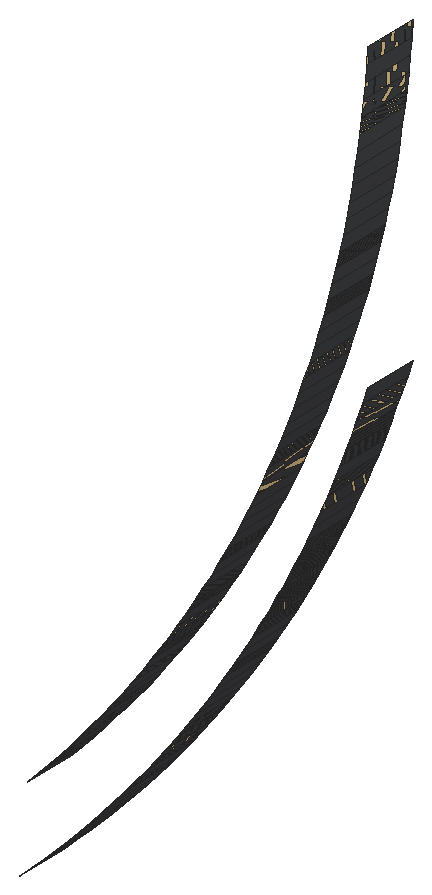
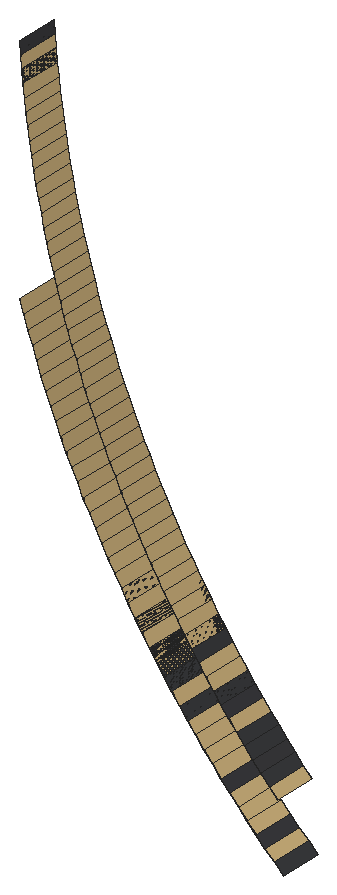
# SketchUp Ruby script. Lengths in inches.
U = 1.inch
M = Sketchup.active_model
def pt(a) = Geom::Point3d.new(a.map { |v| v * U })
def face(e, loops, mat)
  f = e.add_face(loops[0].map { |a| pt(a) })
  loops[1..].each { |l| e.add_face(l.map { |a| pt(a) }).erase! }
  f.material = f.back_material = mat if mat
  f
end
# faces: each face lists its corners as indices into pts; further lists are holes
def faces(e, pts, list, mat = nil) = list.each { |f| face(e, (f[0].is_a?(Array) ? f : [f]).map { |l| l.map { |i| pts[i] } }, mat) }
# xy, xz, yz: faces in a plane at the given z, y or x. An outline is a flat list of corners, or four numbers for a rectangle; further outlines are holes
def ring(l) = l.size == 4 ? [[l[0], l[1]], [l[2], l[1]], [l[2], l[3]], [l[0], l[3]]] : l.each_slice(2).to_a
def flat(e, list, mat, &to3) = list.each { |f| face(e, (f[0].is_a?(Array) ? f : [f]).map { |l| ring(l).map { |u, v| to3.(u, v) } }, mat) }
def xy(e, z, list, mat = nil) = flat(e, list, mat) { |x, y| [x, y, z] }
def xz(e, y, list, mat = nil) = flat(e, list, mat) { |x, z| [x, y, z] }
def yz(e, x, list, mat = nil) = flat(e, list, mat) { |y, z| [x, y, z] }
def lines(e, pts, list) = list.each { |a, b| e.add_line(pt(pts[a]), pt(pts[b])) }
# prism: a flat outline (further loops are holes) pulled along v
def prism(e, loops, v, mat = nil)
  f = face(e, loops, mat); d = Geom::Vector3d.new(v.map { |x| x * U })
  f.pushpull(f.normal.samedirection?(d) ? d.length : -d.length)
end
def box(e, o, s, mat = nil) = prism(e, [[o, [o[0] + s[0], o[1], o[2]], [o[0] + s[0], o[1] + s[1], o[2]], [o[0], o[1] + s[1], o[2]]]], [0, 0, s[2]], mat)
def at(x, y, z, deg = 0) = Geom::Transformation.translation(pt([x, y, z])) * Geom::Transformation.rotation(ORIGIN, Z_AXIS, deg.degrees)
def axes(o, x, y, z) = Geom::Transformation.new([*x, 0, *y, 0, *z, 0, *pt(o).to_a, 1])
def part(name) = M.definitions.add(name)
# library, detail: a bought-in or finely detailed component or shape, given as its bounding box
def library(name, o, s) = part(name).tap { |d| box(d.entities, o, s) }
def detail(e, o, s) = box(e.add_group.entities, o, s)
def put(e, d, t, mat = nil) = e.add_instance(d, t).tap { |i| i.material = mat if mat }
def group(e, t, mat = nil) = e.add_group.tap { |g| g.transformation = t; g.material = mat if mat }.entities
root = M.entities
M.materials.add("1432 AP 8245 TAR ROAD").color = [71, 72, 75]
M.materials.add("Outer Light").color = [251, 217, 152]
p = [[417.09,95.37,295.4],[417.42,95.37,295.72],[417.42,96.87,295.72],[417.09,96.87,295.4],[417.75,95.37,296.04],[417.75,96.87,296.04],
  [417.42,96.87,295.72],[417.75,96.87,296.04],[417.75,95.37,296.04],[417.42,95.37,295.72],[418.07,95.37,296.37],[418.07,96.87,296.37],
  [418.07,96.87,296.37],[418.07,95.37,296.37],[418.39,95.37,296.7],[418.39,96.87,296.7],[418.39,96.87,296.7],[418.39,95.37,296.7],
  [418.7,95.37,297.03],[418.7,96.87,297.03],[418.7,96.87,297.03],[418.7,95.37,297.03],[419.01,95.37,297.37],[419.01,96.87,297.37],
  [419.01,96.87,297.37],[419.01,95.37,297.37],[419.3125,95.37,297.71],[419.3125,96.87,297.71],[419.3125,96.87,297.71],[419.3125,95.37,297.71],
  [417.6,95.37,298.05],[417.3,95.37,297.73],[417.3,96.87,297.73],[417.6,96.87,298.05],[417.6,96.87,298.05],[417.3,96.87,297.73],
  [417.3,95.37,297.73],[417.6,95.37,298.05],[419.61,95.37,298.0625],[419.61,96.87,298.0625],[419.61,96.87,298.0625],[419.61,95.37,298.0625],
  [417.9,95.37,298.375],[417.9,96.87,298.375],[417.9,96.87,298.375],[417.9,95.37,298.375],[419.91,95.37,298.41],[419.91,96.87,298.41],
  [419.91,96.87,298.41],[419.91,95.37,298.41],[418.1875,95.37,298.7],[418.1875,96.87,298.7],[418.1875,96.87,298.7],[418.1875,95.37,298.7],
  [420.2,95.37,298.77],[420.2,96.87,298.77],[420.2,96.87,298.77],[420.2,95.37,298.77],[418.47,95.37,299.04],[418.47,96.87,299.04],
  [418.47,96.87,299.04],[418.47,95.37,299.04],[420.49,95.37,299.125],[420.49,96.87,299.125],[420.49,96.87,299.125],[420.49,95.37,299.125],
  [418.76,95.37,299.37],[418.76,96.87,299.37],[418.76,96.87,299.37],[418.76,95.37,299.37],[420.77,95.37,299.49],[420.77,96.87,299.49],
  [420.77,96.87,299.49],[420.77,95.37,299.49],[419.03,95.37,299.71],[419.03,96.87,299.71],[419.03,96.87,299.71],[419.03,95.37,299.71],
  [421.04,95.37,299.85],[421.04,96.87,299.85],[421.04,96.87,299.85],[421.04,95.37,299.85],[419.31,95.37,300.05],[419.31,96.87,300.05],
  [419.31,96.87,300.05],[419.31,95.37,300.05],[421.32,95.37,300.22],[421.32,96.87,300.22],[421.32,96.87,300.22],[421.32,95.37,300.22],
  [419.58,95.37,300.4],[419.58,96.87,300.4],[419.58,96.87,300.4],[419.58,95.37,300.4],[421.58,95.37,300.59],[421.58,96.87,300.59],
  [421.58,96.87,300.59],[421.58,95.37,300.59],[419.84,95.37,300.75],[419.84,96.87,300.75],[419.84,96.87,300.75],[419.84,95.37,300.75],
  [421.84,95.37,300.97],[421.84,96.87,300.97],[421.84,96.87,300.97],[421.84,95.37,300.97],[420.1,95.37,301.1],[420.1,96.87,301.1],
  [420.1,96.87,301.1],[420.1,95.37,301.1],[422.1,95.37,301.35],[422.1,96.87,301.35],[422.1,96.87,301.35],[422.1,95.37,301.35],
  [420.36,95.37,301.46],[420.36,96.87,301.46],[420.36,96.87,301.46],[420.36,95.37,301.46],[422.35,95.37,301.73],[422.35,96.87,301.73],
  [422.35,96.87,301.73],[422.35,95.37,301.73],[420.61,95.37,301.82],[420.61,96.87,301.82],[420.61,96.87,301.82],[420.61,95.37,301.82],
  [422.6,95.37,302.12],[422.6,96.87,302.12],[422.6,96.87,302.12],[422.6,95.37,302.12],[420.85,95.37,302.18],[420.85,96.87,302.18],
  [420.85,96.87,302.18],[420.85,95.37,302.18],[422.84,95.37,302.5],[422.84,96.87,302.5],[422.84,96.87,302.5],[422.84,95.37,302.5],
  [421.1,95.37,302.55],[421.1,96.87,302.55],[421.1,96.87,302.55],[421.1,95.37,302.55],[421.33,95.37,302.92],[421.33,96.87,302.92],
  [421.33,96.87,302.92],[421.33,95.37,302.92],[423.08,95.37,302.9],[423.08,96.87,302.9],[423.08,96.87,302.9],[423.08,95.37,302.9],
  [421.5625,95.37,303.29],[421.5625,96.87,303.29],[421.5625,96.87,303.29],[421.5625,95.37,303.29],[423.3125,95.37,303.29],[423.3125,96.87,303.29],
  [423.3125,96.87,303.29],[423.3125,95.37,303.29],[421.79,95.37,303.66],[421.79,96.87,303.66],[421.79,96.87,303.66],[421.79,95.37,303.66],
  [423.54,95.37,303.69],[423.54,96.87,303.69],[423.54,96.87,303.69],[423.54,95.37,303.69],[422.01,95.37,304.04],[422.01,96.87,304.04],
  [422.01,96.87,304.04],[422.01,95.37,304.04],[423.76,95.37,304.09],[423.76,96.87,304.09],[423.76,96.87,304.09],[423.76,95.37,304.09],
  [422.23,95.37,304.42],[422.23,96.87,304.42],[422.23,96.87,304.42],[422.23,95.37,304.42],[423.97,95.37,304.5],[423.97,96.87,304.5],
  [423.97,96.87,304.5],[423.97,95.37,304.5],[422.44,95.37,304.81],[422.44,96.87,304.81],[422.44,96.87,304.81],[422.44,95.37,304.81],
  [424.19,95.37,304.9],[424.19,96.87,304.9],[424.19,96.87,304.9],[424.19,95.37,304.9],[422.65,95.37,305.19],[422.65,96.87,305.19],
  [422.65,96.87,305.19],[422.65,95.37,305.19],[424.39,95.37,305.3125],[424.39,96.87,305.3125],[424.39,96.87,305.3125],[424.39,95.37,305.3125],
  [422.85,95.37,305.58],[422.85,96.87,305.58],[422.85,96.87,305.58],[422.85,95.37,305.58],[424.59,95.37,305.72],[424.59,96.87,305.72],
  [424.59,96.87,305.72],[424.59,95.37,305.72],[423.05,95.37,305.98],[423.05,96.87,305.98],[423.05,96.87,305.98],[423.05,95.37,305.98],
  [424.79,95.37,306.14],[424.79,96.87,306.14],[424.79,96.87,306.14],[424.79,95.37,306.14],[423.24,95.37,306.37],[423.24,96.87,306.37],
  [423.24,96.87,306.37],[423.24,95.37,306.37],[424.97,95.37,306.56],[424.97,96.87,306.56],[424.97,96.87,306.56],[424.97,95.37,306.56],
  [423.42,95.37,306.77],[423.42,96.87,306.77],[423.42,96.87,306.77],[423.42,95.37,306.77],[425.16,95.37,306.98],[425.16,96.87,306.98],
  [425.16,96.87,306.98],[425.16,95.37,306.98],[423.6,95.37,307.17],[423.6,96.87,307.17],[423.6,96.87,307.17],[423.6,95.37,307.17],
  [425.34,95.37,307.4],[425.34,96.87,307.4],[425.34,96.87,307.4],[425.34,95.37,307.4],[423.78,95.37,307.57],[423.78,96.87,307.57],
  [423.78,96.87,307.57],[423.78,95.37,307.57],[425.51,95.37,307.82],[425.51,96.87,307.82],[425.51,96.87,307.82],[425.51,95.37,307.82],
  [423.95,95.37,307.97],[423.95,96.87,307.97],[423.95,96.87,307.97],[423.95,95.37,307.97],[425.68,95.37,308.25],[425.68,96.87,308.25],
  [425.68,96.87,308.25],[425.68,95.37,308.25],[424.12,95.37,308.38],[424.12,96.87,308.38],[424.12,96.87,308.38],[424.12,95.37,308.38],
  [425.84,95.37,308.68],[425.84,96.87,308.68],[425.84,96.87,308.68],[425.84,95.37,308.68],[424.27,95.37,308.79],[424.27,96.87,308.79],
  [424.27,96.87,308.79],[424.27,95.37,308.79],[425.99,95.37,309.11],[425.99,96.87,309.11],[425.99,96.87,309.11],[425.99,95.37,309.11],
  [424.43,95.37,309.2],[424.43,96.87,309.2],[424.43,96.87,309.2],[424.43,95.37,309.2],[426.14,95.37,309.54],[426.14,96.87,309.54],
  [426.14,96.87,309.54],[426.14,95.37,309.54],[424.58,95.37,309.61],[424.58,96.87,309.61],[424.58,96.87,309.61],[424.58,95.37,309.61],
  [426.29,95.37,309.98],[426.29,96.87,309.98],[426.29,96.87,309.98],[426.29,95.37,309.98],[424.72,95.37,310.02],[424.72,96.87,310.02],
  [424.72,96.87,310.02],[424.72,95.37,310.02],[424.86,95.37,310.44],[424.86,96.87,310.44],[424.86,96.87,310.44],[424.86,95.37,310.44],
  [426.43,95.37,310.41],[426.43,96.87,310.41],[426.43,96.87,310.41],[426.43,95.37,310.41],[424.99,95.37,310.86],[424.99,96.87,310.86],
  [424.99,96.87,310.86],[424.99,95.37,310.86],[425.12,95.37,311.28],[425.12,96.87,311.28],[425.12,96.87,311.28],[425.12,95.37,311.28],
  [425.24,95.37,311.7],[425.24,96.87,311.7],[425.24,96.87,311.7],[425.24,95.37,311.7],[425.36,95.37,312.12],[425.36,96.87,312.12],
  [425.36,96.87,312.12],[425.36,95.37,312.12],[425.47,95.37,312.55],[425.47,96.87,312.55],[425.47,96.87,312.55],[425.47,95.37,312.55],
  [425.57,95.37,312.97],[425.57,96.87,312.97],[425.57,96.87,312.97],[425.57,95.37,312.97],[425.67,95.37,313.4],[425.67,96.87,313.4],
  [425.67,96.87,313.4],[425.67,95.37,313.4],[425.77,95.37,313.83],[425.77,96.87,313.83],[425.77,96.87,313.83],[425.77,95.37,313.83],
  [425.86,95.37,314.26],[425.86,96.87,314.26],[425.86,96.87,314.26],[425.86,95.37,314.26],[425.9375,95.37,314.6875],[425.9375,96.87,314.6875],
  [425.9375,96.87,314.6875],[425.9375,95.37,314.6875],[426.02,95.37,315.12],[426.02,96.87,315.12],[426.02,96.87,315.12],[426.02,95.37,315.12],
  [426.09,95.37,315.55],[426.09,96.87,315.55],[426.09,96.87,315.55],[426.09,95.37,315.55],[426.15,95.37,315.99],[426.15,96.87,315.99],
  [426.15,96.87,315.99],[426.15,95.37,315.99],[426.21,95.37,316.42],[426.21,96.87,316.42],[426.21,96.87,316.42],[426.21,95.37,316.42],
  [426.27,95.37,316.85],[426.27,96.87,316.85],[426.27,96.87,316.85],[426.27,95.37,316.85],[426.32,95.37,317.29],[426.32,96.87,317.29],
  [426.32,96.87,317.29],[426.32,95.37,317.29],[426.36,95.37,317.73],[426.36,96.87,317.73],[426.36,96.87,317.73],[426.36,95.37,317.73],
  [426.4,95.37,318.16],[426.4,96.87,318.16],[426.4,96.87,318.16],[426.4,95.37,318.16],[426.43,95.37,318.6],[426.43,96.87,318.6],
  [426.43,96.87,318.6],[426.43,95.37,318.6]]
faces(root,p,[[0,1,2,3],[1,4,5,2],[4,10,11,5],[10,14,15,11],[14,18,19,15],[18,22,23,19],[22,26,27,23],[30,31,32,33],
  [26,38,39,27],[42,30,33,43],[38,46,47,39],[50,42,43,51],[46,54,55,47],[58,50,51,59],[54,62,63,55],[66,58,59,67],
  [62,70,71,63],[74,66,67,75],[70,78,79,71],[82,74,75,83],[78,86,87,79],[90,82,83,91],[86,94,95,87],[98,90,91,99],
  [94,102,103,95],[106,98,99,107],[102,110,111,103],[114,106,107,115],[110,118,119,111],[122,114,115,123],[118,126,127,119],[130,122,123,131],
  [126,134,135,127],[138,130,131,139],[142,138,139,143],[134,146,147,135],[150,142,143,151],[146,154,155,147],[158,150,151,159],[154,162,163,155],
  [166,158,159,167],[162,170,171,163],[174,166,167,175],[170,178,179,171],[182,174,175,183],[178,186,187,179],[190,182,183,191],[186,194,195,187],
  [198,190,191,199],[194,202,203,195],[206,198,199,207],[202,210,211,203],[214,206,207,215],[210,218,219,211],[222,214,215,223],[218,226,227,219],
  [230,222,223,231],[226,234,235,227],[238,230,231,239],[234,242,243,235],[246,238,239,247],[242,250,251,243],[254,246,247,255],[250,258,259,251],
  [262,254,255,263],[258,266,267,259],[270,262,263,271],[266,274,275,267],[278,270,271,279],[274,282,283,275],[286,278,279,287],[290,286,287,291],
  [282,294,295,283],[298,290,291,299],[302,298,299,303],[306,302,303,307],[310,306,307,311],[314,310,311,315],[318,314,315,319],[322,318,319,323],
  [326,322,323,327],[330,326,327,331],[334,330,331,335],[338,334,335,339],[342,338,339,343],[346,342,343,347],[350,346,347,351],[354,350,351,355],
  [358,354,355,359],[362,358,359,363],[366,362,363,367],[370,366,367,371]],"1432 AP 8245 TAR ROAD")
faces(root,p,[[6,7,8,9],[7,12,13,8],[12,16,17,13],[16,20,21,17],[20,24,25,21],[24,28,29,25],[34,35,36,37],[28,40,41,29],
  [44,34,37,45],[40,48,49,41],[52,44,45,53],[48,56,57,49],[60,52,53,61],[56,64,65,57],[68,60,61,69],[64,72,73,65],
  [76,68,69,77],[72,80,81,73],[84,76,77,85],[80,88,89,81],[92,84,85,93],[88,96,97,89],[100,92,93,101],[96,104,105,97],
  [108,100,101,109],[104,112,113,105],[116,108,109,117],[112,120,121,113],[124,116,117,125],[120,128,129,121],[132,124,125,133],[128,136,137,129],
  [140,132,133,141],[144,140,141,145],[136,148,149,137],[152,144,145,153],[148,156,157,149],[160,152,153,161],[156,164,165,157],[168,160,161,169],
  [164,172,173,165],[176,168,169,177],[172,180,181,173],[184,176,177,185],[180,188,189,181],[192,184,185,193],[188,196,197,189],[200,192,193,201],
  [196,204,205,197],[208,200,201,209],[204,212,213,205],[216,208,209,217],[212,220,221,213],[224,216,217,225],[220,228,229,221],[232,224,225,233],
  [228,236,237,229],[240,232,233,241],[236,244,245,237],[248,240,241,249],[244,252,253,245],[256,248,249,257],[252,260,261,253],[264,256,257,265],
  [260,268,269,261],[272,264,265,273],[268,276,277,269],[280,272,273,281],[276,284,285,277],[288,280,281,289],[292,288,289,293],[284,296,297,285],
  [300,292,293,301],[304,300,301,305],[308,304,305,309],[312,308,309,313],[316,312,313,317],[320,316,317,321],[324,320,321,325],[328,324,325,329],
  [332,328,329,333],[336,332,333,337],[340,336,337,341],[344,340,341,345],[348,344,345,349],[352,348,349,353],[356,352,353,357],[360,356,357,361],
  [364,360,361,365],[368,364,365,369],[372,368,369,373]],"Outer Light")
